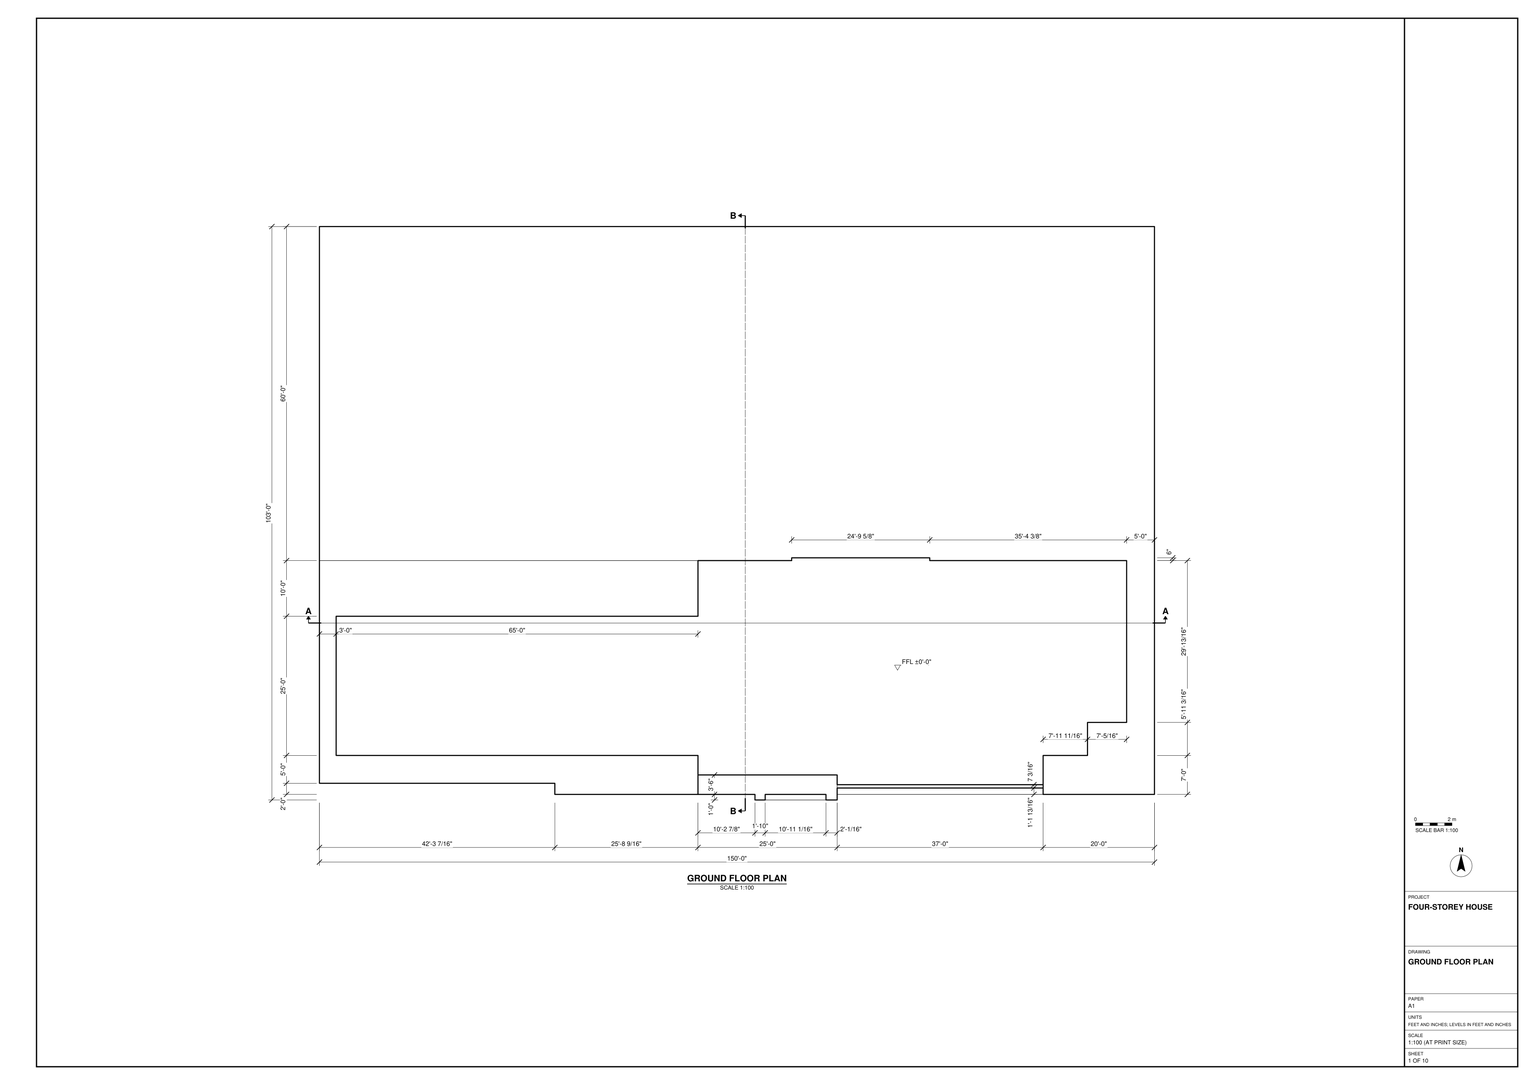
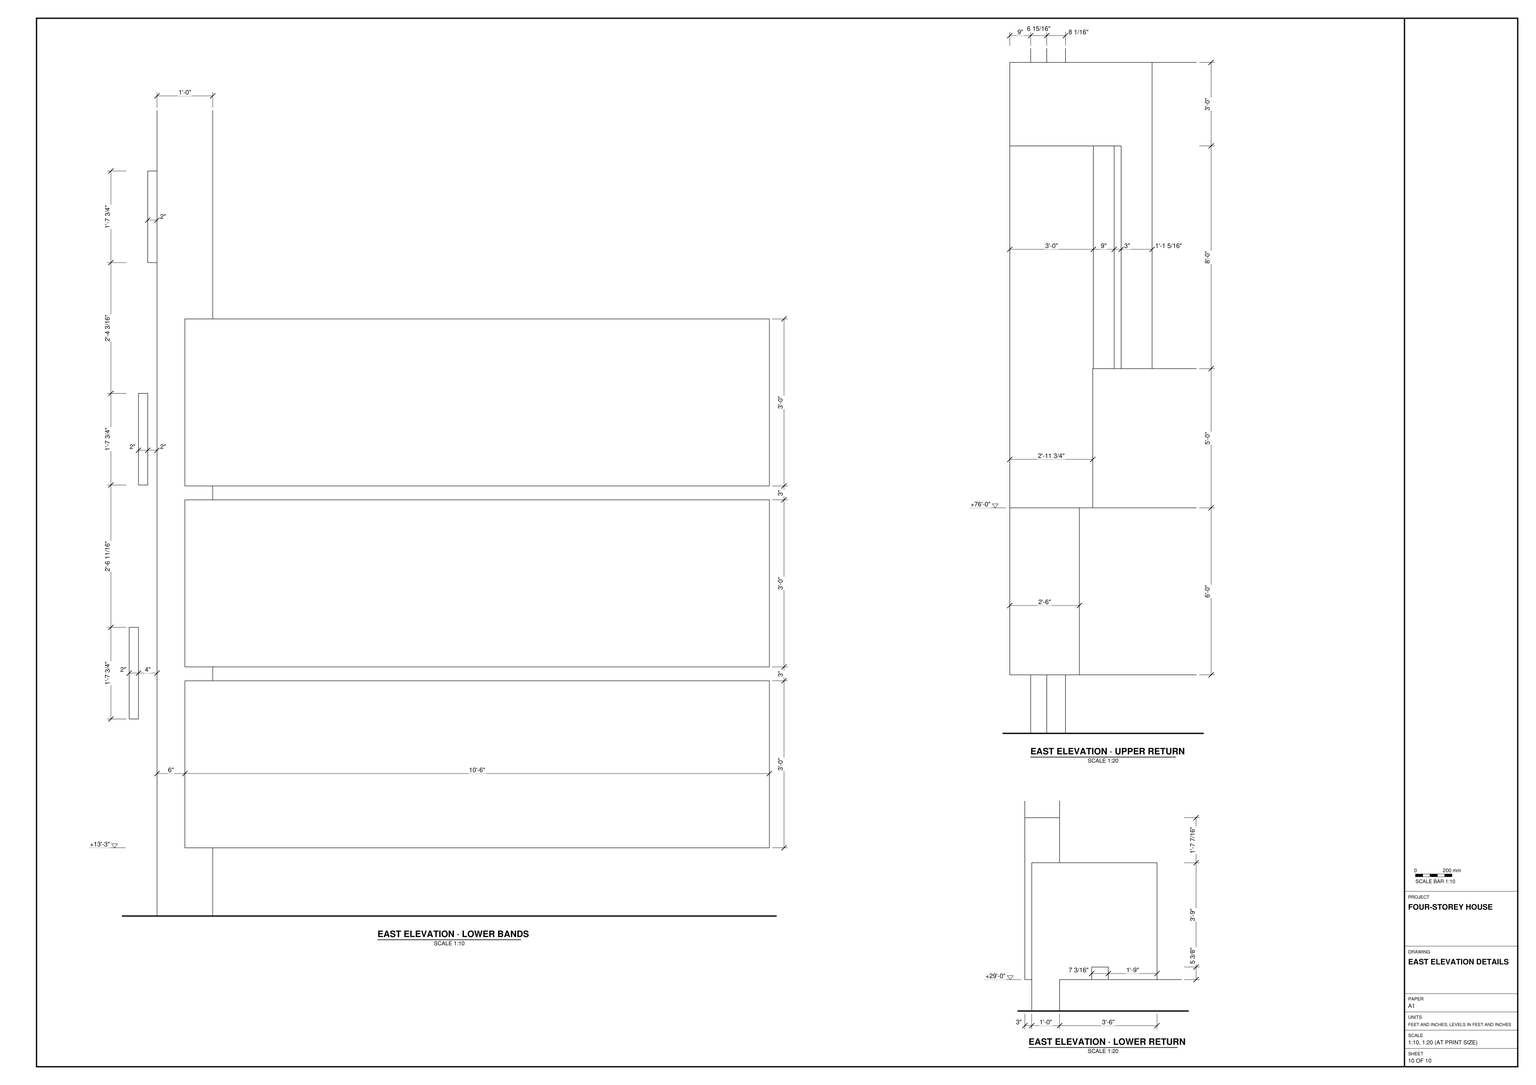
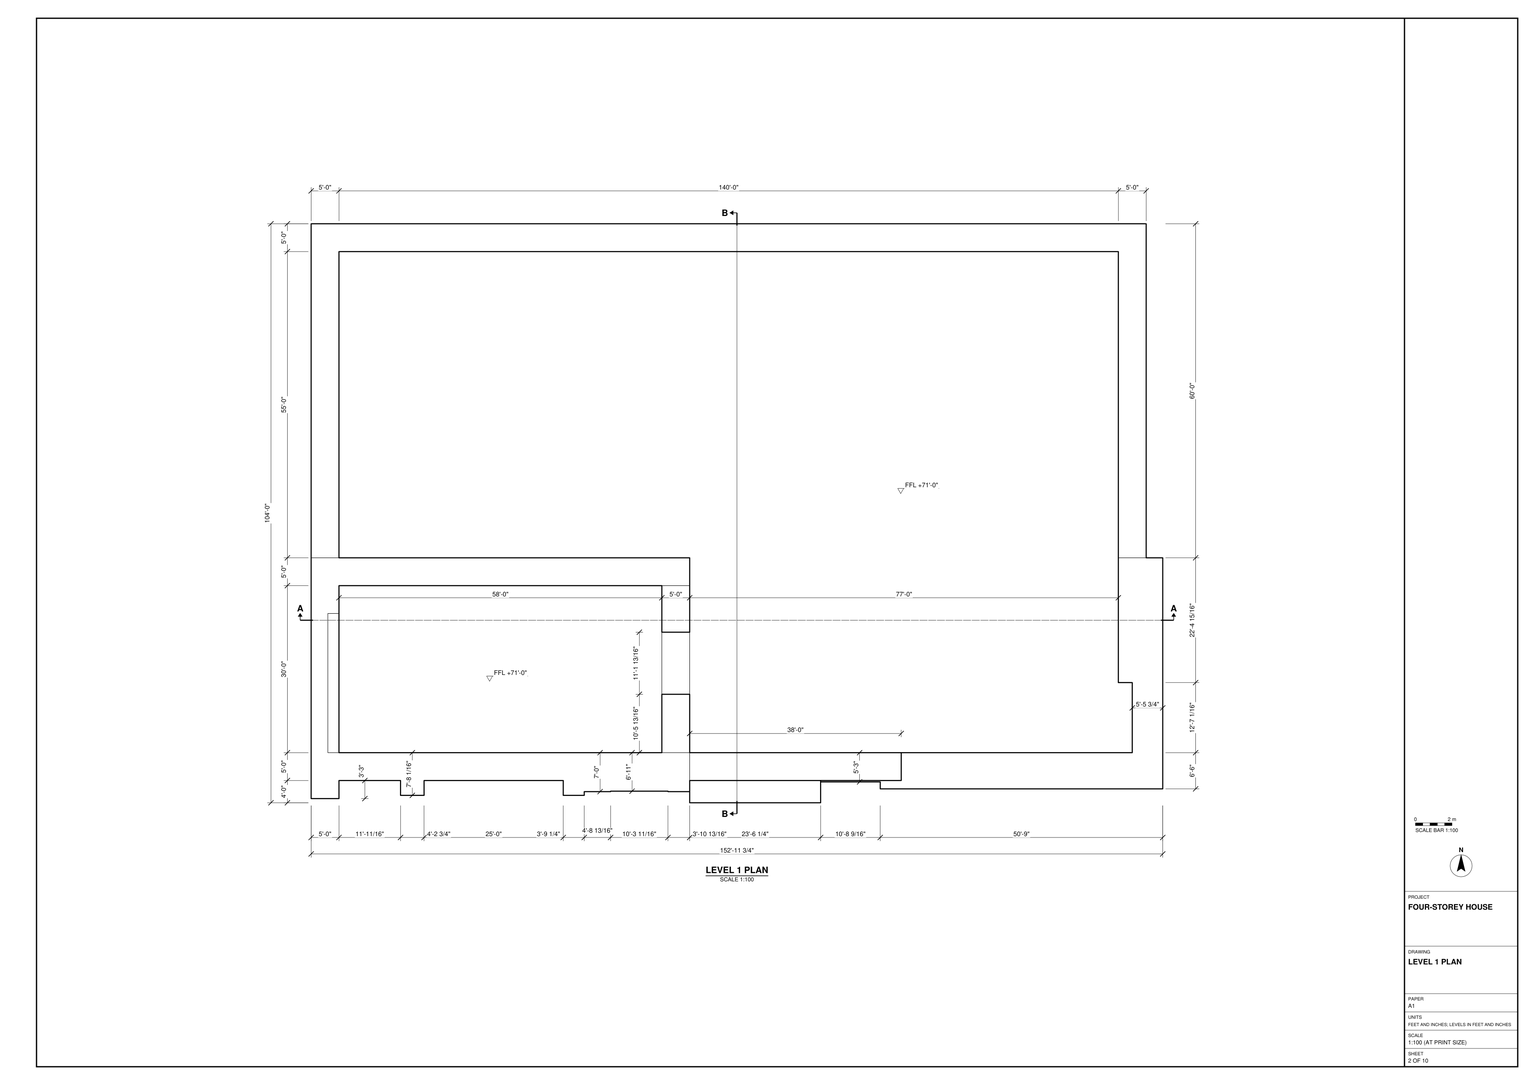
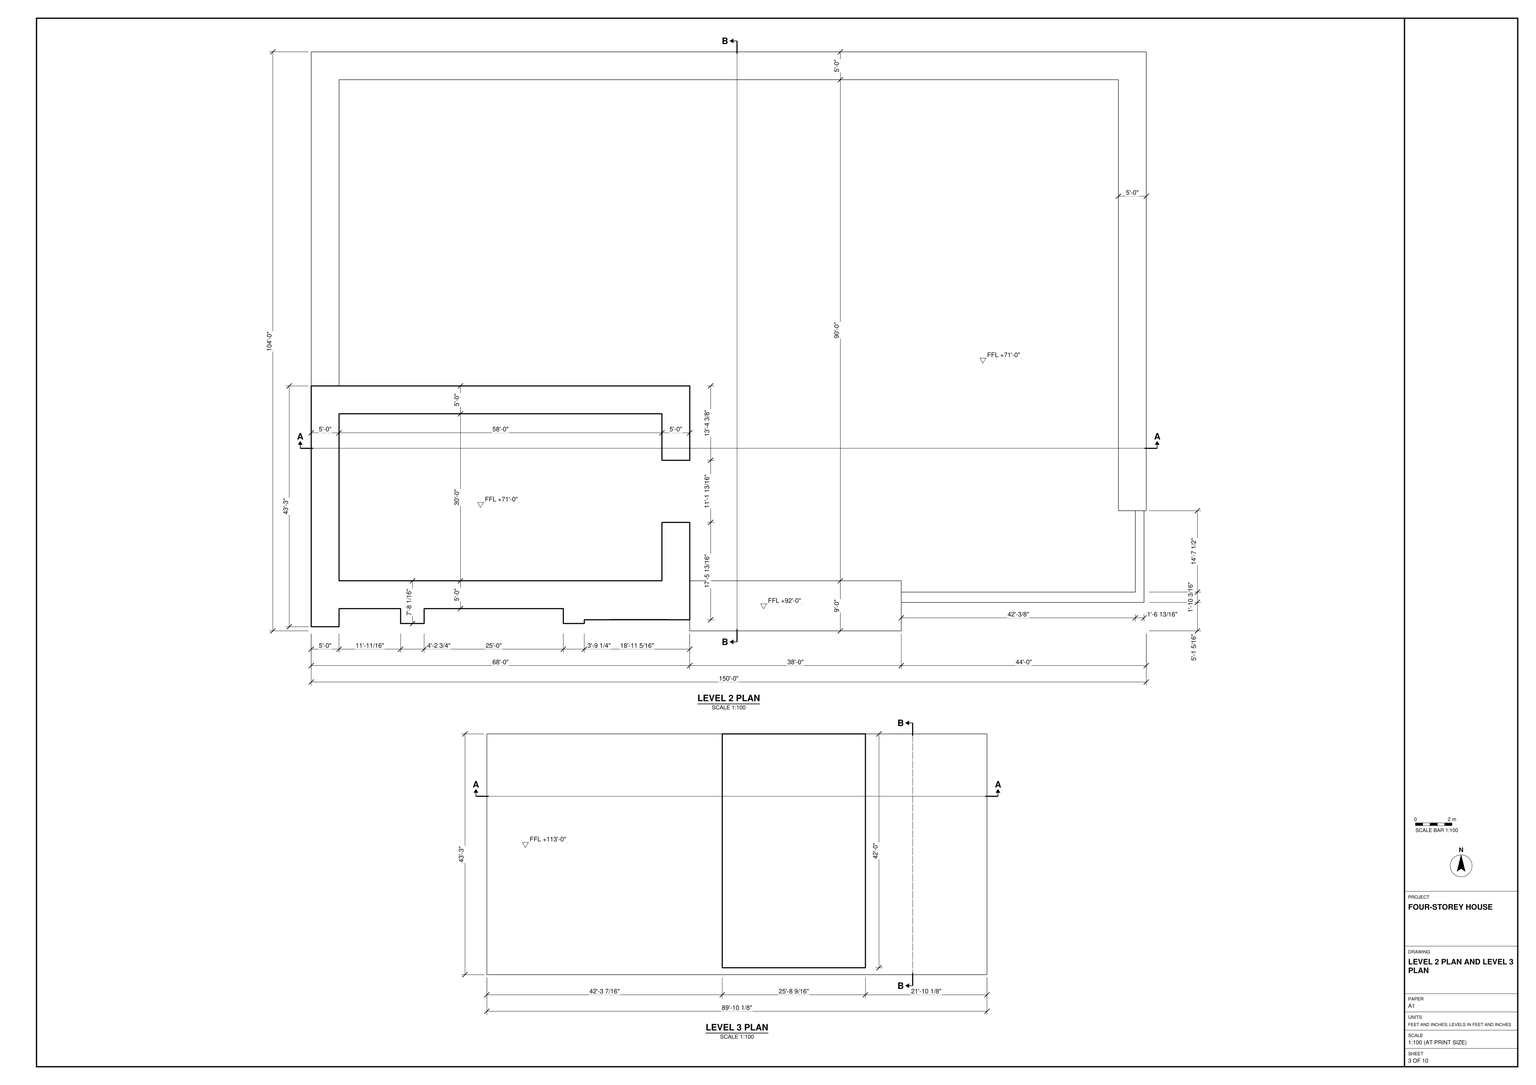
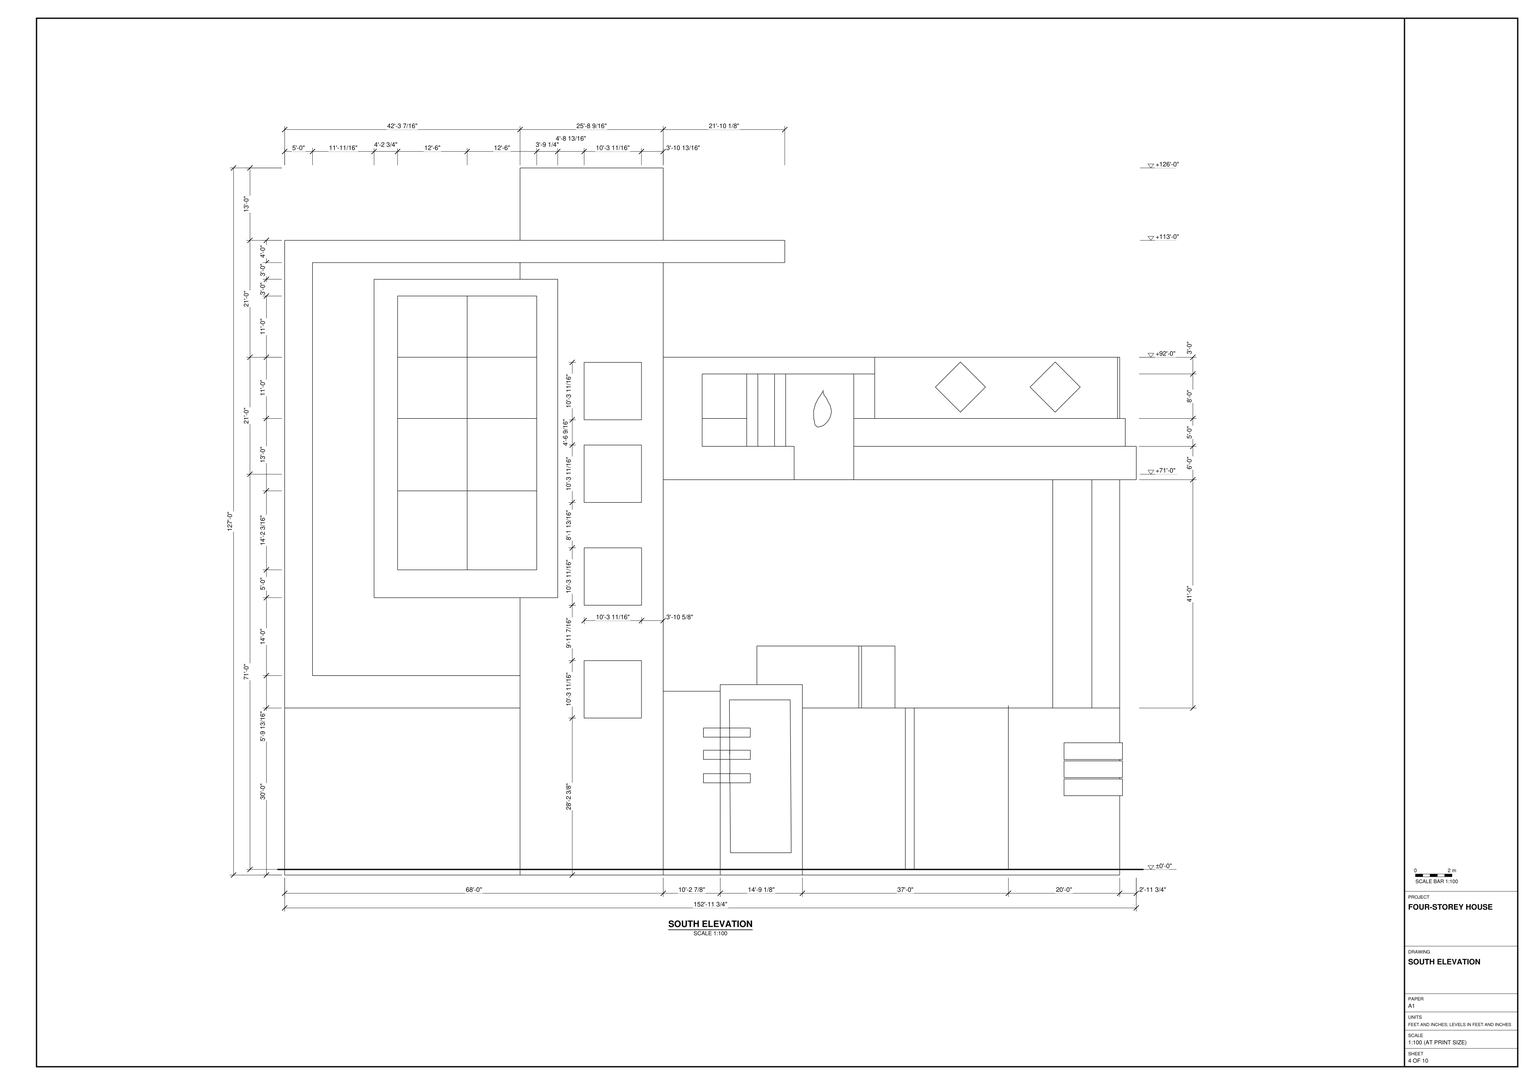
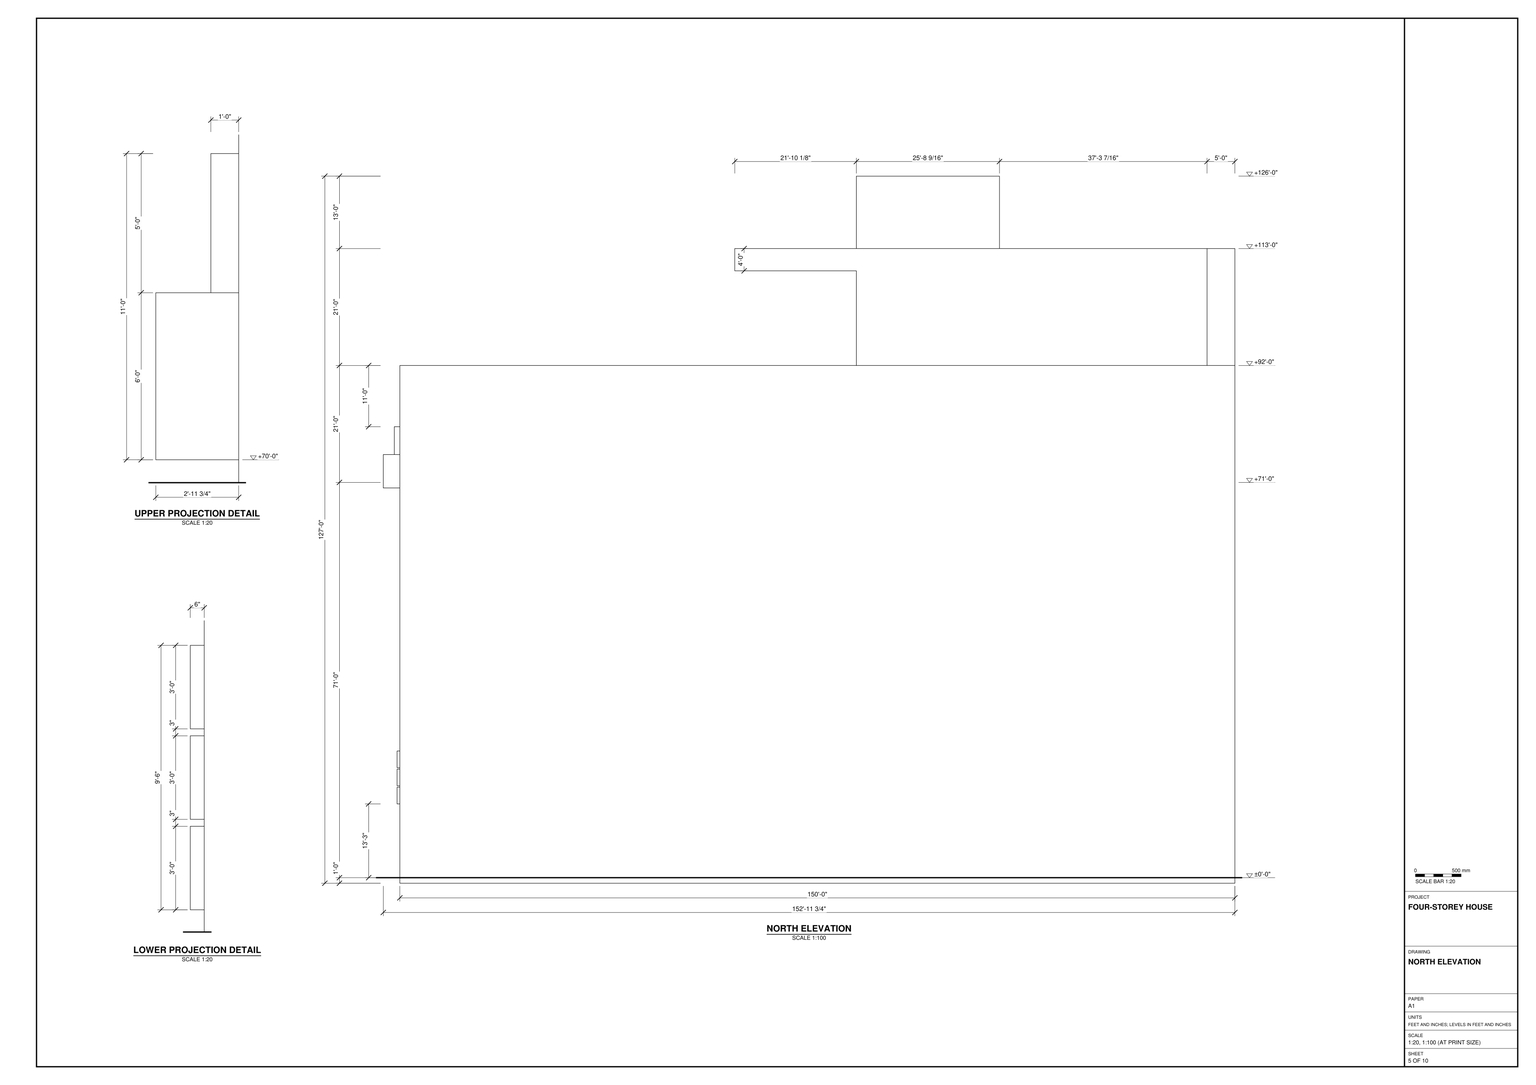
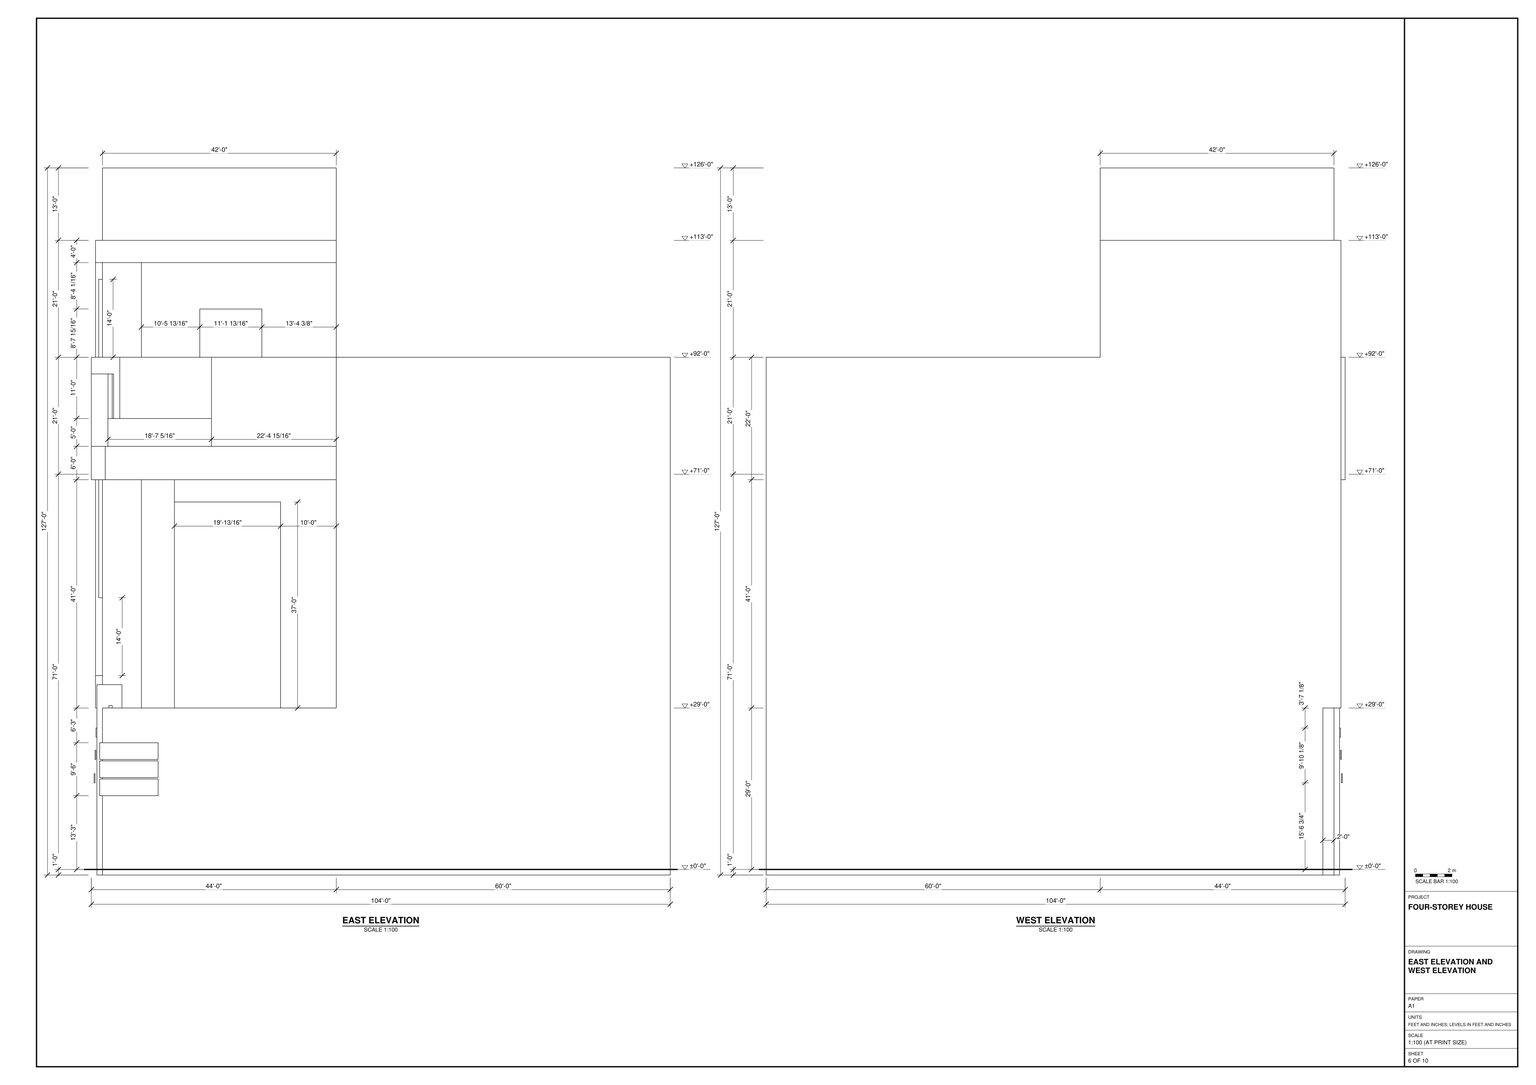
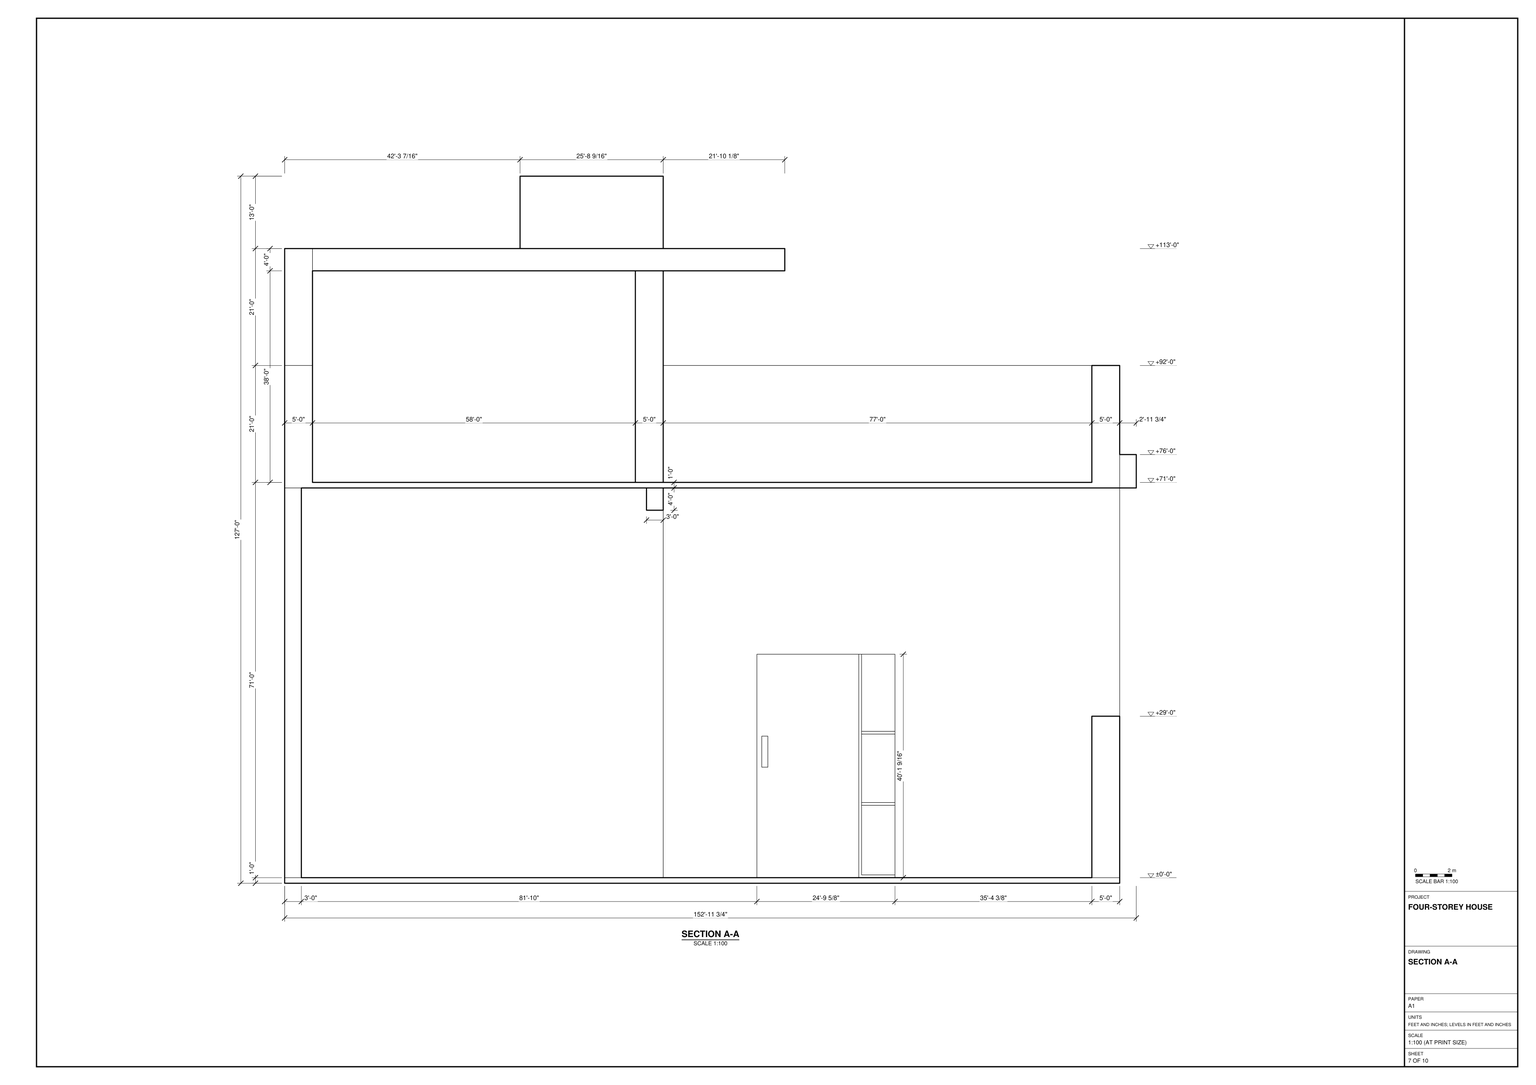
Build the four-storey house in SketchUp using task_files/diagram_01.pdf. Work in feet and inches. The overall model extents are 152'-11 3/4" along X, 104'-0" along Y and 127'-0" along Z. Set the ground floor at ±0'-0" and the three upper floor levels at +71'-0", +92'-0" and +113'-0".

Lay out each floor slab from its own plan. At the ground floor, follow the change in depth between the west and east portions and the stepped outline at the southeast corner. At the first upper level, preserve the relationship between the large L-shaped area and the smaller rectangular area to its southwest. Use the elevations and sections to set the wall profiles, slab edges and roof. Give the walls their drawn thicknesses and include the openings, stairs, built-in joinery and main furniture where shown. On the east elevation, model the three lower horizontal bands with the gaps between them, and follow the detail views for the profiles of the upper and lower returns.

Keep shell elements such as walls, slabs and roof in separate groups or components. Keep each furniture or joinery piece separate and use components for repeated parts. Any decor and loose items shown may be represented by suitable library components. Save one SketchUp model as output_files/four_storey_house_with_its_stepped_east_elevation.skp.

# SketchUp Ruby script. Lengths in inches.
U = 1.inch
M = Sketchup.active_model
def pt(a) = Geom::Point3d.new(a.map { |v| v * U })
def face(e, loops, mat)
  f = e.add_face(loops[0].map { |a| pt(a) })
  loops[1..].each { |l| e.add_face(l.map { |a| pt(a) }).erase! }
  f.material = f.back_material = mat if mat
  f
end
# faces: each face lists its corners as indices into pts; further lists are holes
def faces(e, pts, list, mat = nil) = list.each { |f| face(e, (f[0].is_a?(Array) ? f : [f]).map { |l| l.map { |i| pts[i] } }, mat) }
# xy, xz, yz: faces in a plane at the given z, y or x. An outline is a flat list of corners, or four numbers for a rectangle; further outlines are holes
def ring(l) = l.size == 4 ? [[l[0], l[1]], [l[2], l[1]], [l[2], l[3]], [l[0], l[3]]] : l.each_slice(2).to_a
def flat(e, list, mat, &to3) = list.each { |f| face(e, (f[0].is_a?(Array) ? f : [f]).map { |l| ring(l).map { |u, v| to3.(u, v) } }, mat) }
def xy(e, z, list, mat = nil) = flat(e, list, mat) { |x, y| [x, y, z] }
def xz(e, y, list, mat = nil) = flat(e, list, mat) { |x, z| [x, y, z] }
def yz(e, x, list, mat = nil) = flat(e, list, mat) { |y, z| [x, y, z] }
def lines(e, pts, list) = list.each { |a, b| e.add_line(pt(pts[a]), pt(pts[b])) }
# prism: a flat outline (further loops are holes) pulled along v
def prism(e, loops, v, mat = nil)
  f = face(e, loops, mat); d = Geom::Vector3d.new(v.map { |x| x * U })
  f.pushpull(f.normal.samedirection?(d) ? d.length : -d.length)
end
def box(e, o, s, mat = nil) = prism(e, [[o, [o[0] + s[0], o[1], o[2]], [o[0] + s[0], o[1] + s[1], o[2]], [o[0], o[1] + s[1], o[2]]]], [0, 0, s[2]], mat)
def at(x, y, z, deg = 0) = Geom::Transformation.translation(pt([x, y, z])) * Geom::Transformation.rotation(ORIGIN, Z_AXIS, deg.degrees)
def axes(o, x, y, z) = Geom::Transformation.new([*x, 0, *y, 0, *z, 0, *pt(o).to_a, 1])
def part(name) = M.definitions.add(name)
# library, detail: a bought-in or finely detailed component or shape, given as its bounding box
def library(name, o, s) = part(name).tap { |d| box(d.entities, o, s) }
def detail(e, o, s) = box(e.add_group.entities, o, s)
def put(e, d, t, mat = nil) = e.add_instance(d, t).tap { |i| i.material = mat if mat }
def group(e, t, mat = nil) = e.add_group.tap { |g| g.transformation = t; g.material = mat if mat }.entities
root = M.entities
M.materials.add("[0026_LightSalmon]").color = [255, 160, 122]
M.materials.add("[0029_BlanchedAlmond]").color = [209, 192, 168]
M.materials.add("[0030_OldLace]").color = [253, 245, 230]
M.materials.add("[0047_Khaki]").color = [201, 193, 117]
M.materials.add("[0058_Olive]").color = [76, 76, 0]
M.materials.add("[0119_RosyBrown]").color = [76, 58, 58]
M.materials.add("[0136_Charcoal]").color = [35, 35, 35]
M.materials.add("[0137_Black]").color = [0, 0, 0]
M.materials.add("[Blacktop Old 01]").color = [132, 136, 139]
M.materials.add("[Cladding Siding Tan]").color = [165, 128, 97]
M.materials.add("[Granite Brown]").color = [126, 104, 91]
M.materials.add("[Stone Flagstone Ashlar]").color = [175, 116, 102]
M.materials.add("[Stone Marble]").color = [143, 138, 136]
M.materials.add("[Translucent Glass Blue]").color = [100, 149, 237]
M.materials["[Translucent Glass Blue]"].alpha = 0.5
M.materials.add("[Translucent Glass Gray]").color = [128, 128, 128]
M.materials["[Translucent Glass Gray]"].alpha = 0.5
xy(root,0,[[938.875,12,938.875,24,507.4375,24,507.4375,48,0,48,0,1248,1800,1248,1800,24,1116,24,1116,12]])
xy(root,12,[[1116,24,1560,37.83],[1116,37.83,1560,45]])
xy(root,12,[[1116,45,1560,45,1560,108,1655.6875,108,1655.6875,179.1875,1740,179.1875,1740,528,1315.61,528,1315.61,534,1017.99,534,1017.99,528,816,528,816,408,36,408,36,108,816,108,816,66,1116,66]],"[Granite Brown]")
xy(root,48,[[960.9375,12,1092,24]],"[Blacktop Old 01]")
xy(root,171,[[1680,18,1806,24],[1800,24,1806,144]],"[Blacktop Old 01]")
xy(root,198.76,[[902.7,6,938.875,8],[938.875,6,959.26,8],[959.26,6,1003.82,8]],"[0047_Khaki]")
xy(root,207,[[1680,18,1806,24],[1800,24,1806,144]],"[0058_Olive]")
xy(root,210,[[1680,18,1806,24],[1800,24,1806,144]],"[Blacktop Old 01]")
xy(root,218.51,[[1003.6875,6,1003.82,8]])
xy(root,218.51,[[902.7,6,938.875,8],[938.875,6,959.125,8],[959.26,6,1003.6875,8]],"[0047_Khaki]")
xy(root,246,[[1680,18,1806,24],[1800,24,1806,144]],"[0058_Olive]")
xy(root,249,[[1680,18,1800,24],[1800,18,1806,144]],"[Blacktop Old 01]")
xy(root,249.2,[[902.7,8,938.875,10],[938.875,8,959.26,10],[959.26,8,1003.82,10]],"[0047_Khaki]")
xy(root,268.95,[[1003.6875,8,1003.82,10]])
xy(root,268.95,[[902.7,8,938.875,10],[938.875,8,959.125,10],[959.26,8,1003.6875,10]],"[0047_Khaki]")
xy(root,285,[[1680,18,1800,24],[1800,18,1806,144]],"[0058_Olive]")
xy(root,297.14,[[902.7,10,938.875,12],[938.875,10,959.26,12],[959.26,10,1003.82,12]],"[0047_Khaki]")
xy(root,316.89,[[1003.6875,10,1003.82,12]])
xy(root,316.89,[[902.7,10,938.875,12],[938.875,10,959.125,12],[959.26,10,1003.6875,12]],"[0047_Khaki]")
xy(root,338.36,[[645.5,24,769.18,25]])
xy(root,360,[[0,9,507.4375,48],[1560,24,1800,24,1800,528,1740,528,1740,108,1560,108],[1116,37.83,1560,45]])
xy(root,377.47,[[958.72,12,1089.78,24]],"[Blacktop Old 01]")
xy(root,396,[[816,24,938.875,66]])
xy(root,410.375,[[938.875,12,1116,66]],"[0058_Olive]")
xy(root,429.79,[[60,9,507.4375,48]],"[Blacktop Old 01]")
xy(root,462.04,[[645.5,24,769.18,25]])
xy(root,493.57,[[1017.99,528,1315.61,534]],"[0136_Charcoal]")
xy(root,581.5,[[645.66,24,769.35,25]])
xy(root,597.79,[[192.6875,15.9375,192.6875,48,507.4375,48,507.4375,24,588.6875,24,588.6875,15.9375]],"[0058_Olive]")
xy(root,657.79,[[243.4375,15.9375,543.4375,48]],"[0058_Olive]")
xy(root,705.1875,[[645.66,24,769.35,25]])
xy(root,803.01,[[645.5,24,769.18,25]])
xy(root,804,[[780,108,816,408]],"[Stone Flagstone Ashlar]")
xy(root,852,[[[1226.76,30,1226.76,45,1098.22,45,1098.22,48,816,48,816,528,1835.75,528,1835.75,30],[1655.6875,108,1740,179.1875],[1024.9,157.24,1031.11,158.0625,1036.9,160.46,1041.87,164.27,1045.6875,169.24,1048.08,175.03,1048.9,181.24,1048.08,187.46,1045.6875,193.24,1041.87,198.21,1036.9,202.03,1031.11,204.43,1024.9,205.24,1018.69,204.43,1012.9,202.03,1007.93,198.21,1004.12,193.24,1001.72,187.46,1000.9,181.24,1001.72,175.03,1004.12,169.24,1007.93,164.27,1012.9,160.46,1018.69,158.0625],[1293.34,157.24,1299.55,158.0625,1305.34,160.46,1310.31,164.27,1314.125,169.24,1316.52,175.03,1317.34,181.24,1316.52,187.46,1314.125,193.24,1310.31,198.21,1305.34,202.03,1299.55,204.43,1293.34,205.24,1287.13,204.43,1281.34,202.03,1276.37,198.21,1272.56,193.24,1270.16,187.46,1269.34,181.24,1270.16,175.03,1272.56,169.24,1276.37,164.27,1281.34,160.46,1287.13,158.0625],[1510.65,157.24,1516.86,158.0625,1522.65,160.46,1527.62,164.27,1531.4375,169.24,1533.83,175.03,1534.65,181.24,1533.83,187.46,1531.4375,193.24,1527.62,198.21,1522.65,202.03,1516.86,204.43,1510.65,205.24,1504.44,204.43,1498.65,202.03,1493.68,198.21,1489.87,193.24,1487.47,187.46,1486.65,181.24,1487.47,175.03,1489.87,169.24,1493.68,164.27,1498.65,160.46,1504.44,158.0625]],[780,108,816,408],[1024.9,157.24,1018.69,158.0625,1012.9,160.46,1007.93,164.27,1004.12,169.24,1001.72,175.03,1000.9,181.24,1001.72,187.46,1004.12,193.24,1007.93,198.21,1012.9,202.03,1018.69,204.43,1024.9,205.24,1031.11,204.43,1036.9,202.03,1041.87,198.21,1045.6875,193.24,1048.08,187.46,1048.9,181.24,1048.08,175.03,1045.6875,169.24,1041.87,164.27,1036.9,160.46,1031.11,158.0625],[1293.34,157.24,1287.13,158.0625,1281.34,160.46,1276.37,164.27,1272.56,169.24,1270.16,175.03,1269.34,181.24,1270.16,187.46,1272.56,193.24,1276.37,198.21,1281.34,202.03,1287.13,204.43,1293.34,205.24,1299.55,204.43,1305.34,202.03,1310.31,198.21,1314.125,193.24,1316.52,187.46,1317.34,181.24,1316.52,175.03,1314.125,169.24,1310.31,164.27,1305.34,160.46,1299.55,158.0625],[1510.65,157.24,1504.44,158.0625,1498.65,160.46,1493.68,164.27,1489.87,169.24,1487.47,175.03,1486.65,181.24,1487.47,187.46,1489.87,193.24,1493.68,198.21,1498.65,202.03,1504.44,204.43,1510.65,205.24,1516.86,204.43,1522.65,202.03,1527.62,198.21,1531.4375,193.24,1533.83,187.46,1534.65,181.24,1533.83,175.03,1531.4375,169.24,1527.62,164.27,1522.65,160.46,1516.86,158.0625]])
xy(root,852,[[816,0,1098.22,48]],"[0047_Khaki]")
xy(root,852,[[36,108,780,408]],"[Stone Flagstone Ashlar]")
xy(root,864,[[816,48,1272,108],[60,108,756,468],[756,108,816,233.83],[756,233.83,816,367.65],[756,367.65,816,468]])
xy(root,864,[[816,108,1770,108,1770,259.04,1740,259.04,1740,1188,60,1188,60,528,816,528]],"[0029_BlanchedAlmond]")
xy(root,912,[[1272,48,1800,48,1800,259.04,1795.23,259.04,1795.23,61.34,1272,61.34]])
xy(root,912,[[1272,83.56,1776.4,83.56,1776.4,259.04,1770,259.04,1770,108,1272,108]],"[0029_BlanchedAlmond]")
xy(root,924,[[996,36,1020,48],[1056,36,1080,48],[1020,45,1056,48],[1080,45,1098.22,48],[900,48,996,48.5]])
xy(root,924,[[900,0,1098.22,0,1098.22,45,1080,45,1080,36,1056,36,1056,45,1020,45,1020,36,996,36,996,48,900,48],[1226.76,30,1835.75,30,1835.75,528,1800,528,1800,259.04,1812,259.04,1812,35.75,1226.76,35.75]],"[0047_Khaki]")
xy(root,926.7,[[645.5,24,769.18,25]])
xy(root,981.26,[[645.5,24,769.18,25]])
xy(root,984,[[900,48,996,48.5]])
xy(root,984,[[1226.76,35.75,1812,35.75,1812,259.04,1800,259.04,1800,48,1226.76,48]],"[0026_LightSalmon]")
xy(root,1080,[[996,36,1020,48],[1056,36,1080,48],[1020,45,1056,48],[1080,45,1226.76,48]])
xy(root,1080,[[900,0,900,48,996,48,996,36,1020,36,1020,45,1056,45,1056,36,1080,36,1080,45,1226.76,45,1226.76,48,1272,48,1272,0]],"[0047_Khaki]")
xy(root,1104.94,[[645.5,24,769.18,25]])
xy(root,1116,[[1272,61.34,1795.23,61.34,1795.23,259.04,1776.4,259.04,1776.4,83.56,1272,83.56],[1740,259.04,1800,259.04,1800,1248,0,1248,0,528,60,528,60,1188,1740,1188]],"[0029_BlanchedAlmond]")
xy(root,1116,[[816,0,1272,108]],"[0047_Khaki]")
xy(root,1219.9375,[[756,233.83,816,367.65]])
xy(root,1248,[[243.4375,15.9375,543.4375,48]],"[0058_Olive]")
xy(root,1284,[[192.6875,15.9375,588.6875,15.9375,588.6875,24,507.4375,24,507.4375,48,192.6875,48]],"[0058_Olive]")
xy(root,1320,[[[816,9,1078.125,108],[966.1,34.06,972.25,35.25,977.89,37.99,982.62,42.09,986.13,47.28,988.18,53.2,988.62,59.45,987.43,65.6,984.69,71.24,980.59,75.97,975.4,79.48,969.48,81.53,963.23,81.97,957.08,80.78,951.44,78.04,946.71,73.9375,943.2,68.75,941.15,62.83,940.71,56.58,941.9,50.43,944.64,44.79,948.74,40.06,953.93,36.55,959.85,34.5]],[966.1,34.06,959.85,34.5,953.93,36.55,948.74,40.06,944.64,44.79,941.9,50.43,940.71,56.58,941.15,62.83,943.2,68.75,946.71,73.9375,951.44,78.04,957.08,80.78,963.23,81.97,969.48,81.53,975.4,79.48,980.59,75.97,984.69,71.24,987.43,65.6,988.62,59.45,988.18,53.2,986.13,47.28,982.62,42.09,977.89,37.99,972.25,35.25],[60,108,756,468],[756,108,816,468],[[816,108,1078.125,468],[844.55,155.55,1032.24,184.18],[844.55,222.55,1032.24,251.18],[844.55,284.61,1032.24,313.24],[844.55,347.05,1032.24,375.68],[844.55,410.43,1032.24,439.05]],
  [[816,468,1078.125,528],[966.1,475.68,972.25,476.87,977.89,479.61,982.62,483.71,986.13,488.9,988.18,494.83,988.62,501.08,987.43,507.23,984.69,512.86,980.59,517.6,975.4,521.1,969.48,523.15,963.23,523.6,957.08,522.41,951.44,519.67,946.71,515.5625,943.2,510.375,941.15,504.45,940.71,498.2,941.9,492.05,944.64,486.42,948.74,481.68,953.93,478.17,959.85,476.125]],[966.1,475.68,959.85,476.125,953.93,478.17,948.74,481.68,944.64,486.42,941.9,492.05,940.71,498.2,941.15,504.45,943.2,510.375,946.71,515.5625,951.44,519.67,957.08,522.41,963.23,523.6,969.48,523.15,975.4,521.1,980.59,517.6,984.69,512.86,987.43,507.23,988.62,501.08,988.18,494.83,986.13,488.9,982.62,483.71,977.89,479.61,972.25,476.87]])
xy(root,1320,[[844.55,155.55,1032.24,184.18],[844.55,222.55,1032.24,251.18],[844.55,284.61,1032.24,313.24],[844.55,347.05,1032.24,375.68],[844.55,410.43,1032.24,439.05]],"[0058_Olive]")
xy(root,1320,[[60,9,60,48,507.4375,48,507.4375,24,816,24,816,9]],"[Blacktop Old 01]")
xy(root,1368,[[507.4375,24,816,528]])
xy(root,1368,[[0,9,1078.125,9,1078.125,528,816,528,816,24,507.4375,24,507.4375,528,0,528]],"[0029_BlanchedAlmond]")
xy(root,1524,[[507.4375,24,816,528]],"[Stone Flagstone Ashlar]")
xz(root,0,[[816,852,1098.22,852,1098.22,924,900,924,900,1080,1272,1080,1272,1116,816,1116]],"[0047_Khaki]")
xz(root,6,[[902.7,198.76,938.875,218.51],[938.875,198.76,959.26,198.76,959.125,218.51,938.875,218.51],[959.26,198.76,1003.82,218.51]],"[0047_Khaki]")
xz(root,8,[[902.7,198.76,938.875,218.51],[938.875,198.76,938.875,218.51,959.125,218.51,959.26,198.76],[959.26,198.76,1003.82,218.51]])
xz(root,8,[[902.7,249.2,938.875,268.95],[938.875,249.2,959.26,249.2,959.125,268.95,938.875,268.95],[959.26,249.2,1003.82,268.95]],"[0047_Khaki]")
xz(root,9,[[0,360,507.4375,360,507.4375,429.79,60,429.79,60,1320,1078.125,1320,1078.125,1368,0,1368]],"[Blacktop Old 01]")
xz(root,10,[[902.7,249.2,938.875,268.95],[938.875,249.2,938.875,268.95,959.125,268.95,959.26,249.2],[959.26,249.2,1003.82,268.95]])
xz(root,10,[[902.7,297.14,938.875,316.89],[938.875,297.14,959.26,297.14,959.125,316.89,938.875,316.89],[959.26,297.14,1003.82,316.89]],"[0047_Khaki]")
xz(root,12,[[902.7,297.14,938.875,316.89],[938.875,297.14,938.875,316.89,959.125,316.89,959.26,297.14],[959.26,297.14,959.26,316.89,959.125,316.89],[959.26,297.14,1003.82,316.89]])
xz(root,12,[[938.875,0,1116,0,1116,410.375,938.875,410.375,938.875,316.89,959.125,316.89,958.72,377.47,1089.78,377.47,1092,48,960.9375,48,959.26,297.14,938.875,297.14]],"[0058_Olive]")
xz(root,15.9375,[[[192.6875,597.79,588.6875,1284],[243.4375,657.79,543.4375,1248]]],"[0058_Olive]")
xz(root,18,[[1680,171,1806,207],[1680,210,1806,246],[1680,249,1806,285]],"[0058_Olive]")
xz(root,24,[[1680,249,1800,285]])
xz(root,24,[[816,0,938.875,12],[1116,0,1800,0,1800,171,1680,171,1680,207,1800,207,1800,210,1680,210,1680,246,1800,246,1800,249,1680,249,1680,285,1800,285,1800,360,1560,360,1560,12,1116,12],[816,12,938.875,396],[960.9375,48,1092,48,1089.78,377.47,958.72,377.47]],"[0029_BlanchedAlmond]")
xz(root,24,[[[507.4375,0,816,0,816,1320,507.4375,1320,507.4375,1284,588.6875,1284,588.6875,597.79,507.4375,597.79],[645.5,803.01,769.18,926.7],[645.66,581.5,769.35,705.1875],[645.5,338.36,769.18,462.04],[645.5,981.26,769.18,1104.94]],[507.4375,1368,816,1524]],"[Stone Flagstone Ashlar]")
xz(root,25,[[645.5,338.36,769.18,462.04],[645.66,581.5,769.35,705.1875],[645.5,803.01,769.18,926.7],[645.5,981.26,769.18,1104.94]])
xz(root,30,[[1226.76,852,1835.75,924]],"[0047_Khaki]")
xz(root,35.75,[[1226.76,924,1812,984]],"[0026_LightSalmon]")
xz(root,36,[[996,924,1020,1080],[1056,924,1080,1080]],"[0058_Olive]")
xz(root,37.83,[[1338,12,1357.125,360]],"[0137_Black]")
xz(root,37.83,[[1116,12,1338,360],[1357.125,12,1560,360]],"[Cladding Siding Tan]")
xz(root,45,[[1116,12,1560,360]])
xz(root,45,[[1020,924,1056,1080]],"[0029_BlanchedAlmond]")
xz(root,45,[[1148.98,965.29,1155.99,967.1,1159.14,968,1161.29,969.05,1163.43,970.8,1165.51,972.6,1167.52,974.44,1169.45,976.36,1171.03,978.63,1172.54,980.9,1173.95,983.2,1175.28,985.55,1176.2,987.91,1176.81,990.32,1177.62,993.31,1178.04,995.625,1178.57,997.98,1178.4375,1000.625,1178.18,1003,1177.33,1005.38,1176.97,1007.82,1176.23,1010.83,1175.34,1013.21,1173.89,1015.58,1172.59,1018.22,1170.78,1021.1,1170.22,1022.86,1167.6,1028.03,1162.8,1034.4,1160.35,1042.71,1159.09,1040.51,1157.58,1038.3,1156.34,1036.12,1154.82,1034.24,1153.85,1031.96,1152.26,1029.73,1150.73,1027.74,1149.25,1025.13,1148.08,1022.85,1146.98,1020.57,1145.85,1018.28,1144.28,1015.97,1143.94,1013.61,1142.99,1011.24,1142.36,1008.81,1141.77,1006.06,1140.9375,1003.62,1140.24,1000.85,1140.22,998.1,1140.21,995.65,1140.22,992.88,1140.25,990.16,1140.37,987.71,1140.54,984.95,1140.73,982.53,1141.62,979.57,1142.25,976.86,1142,974.92,1143.57,969.82]],"[0030_OldLace]")
xz(root,45,[[[1098.22,852,1226.76,852,1226.76,1080,1080,1080,1080,924,1098.22,924],[1148.98,965.29,1143.57,969.82,1142,974.92,1142.25,976.86,1141.62,979.57,1140.73,982.53,1140.54,984.95,1140.37,987.71,1140.25,990.16,1140.22,992.88,1140.21,995.65,1140.22,998.1,1140.24,1000.85,1140.9375,1003.62,1141.77,1006.06,1142.36,1008.81,1142.99,1011.24,1143.94,1013.61,1144.28,1015.97,1145.85,1018.28,1146.98,1020.57,1148.08,1022.85,1149.25,1025.13,1150.73,1027.74,1152.26,1029.73,1153.85,1031.96,1154.82,1034.24,1156.34,1036.12,1157.58,1038.3,1159.09,1040.51,1160.35,1042.71,1162.8,1034.4,1167.6,1028.03,1170.22,1022.86,1170.78,1021.1,1172.59,1018.22,1173.89,1015.58,1175.34,1013.21,1176.23,1010.83,1176.97,1007.82,1177.33,1005.38,1178.18,1003,1178.4375,1000.625,1178.57,997.98,1178.04,995.625,1177.62,993.31,1176.81,990.32,1176.2,987.91,1175.28,985.55,1173.95,983.2,1172.54,980.9,1171.03,978.63,1169.45,976.36,1167.52,974.44,1165.51,972.6,1163.43,970.8,1161.29,969.05,1159.14,968,1155.99,967.1]]],"[0058_Olive]")
xz(root,48,[[816,864,1098.22,864,1098.22,924,900,924,900,984,816,984],[1098.22,864,1272,864,1272,984,996,984,996,924,1098.22,924],[1272,912,1800,984]])
xz(root,48,[[60,429.79,507.4375,429.79,507.4375,597.79,192.6875,597.79,192.6875,1284,507.4375,1284,507.4375,1320,60,1320],[900,924,996,984],[900,984,996,1080],[1226.76,984,1272,1080]],"[0029_BlanchedAlmond]")
xz(root,48,[[0,0,507.4375,360]],"[0047_Khaki]")
xz(root,48,[[243.4375,657.79,393.4375,828],[393.4375,657.79,543.4375,828],[243.4375,828,393.4375,984],[393.4375,828,543.4375,984],[243.4375,984,393.4375,1116],
  [393.4375,984,543.4375,1116],[243.4375,1116,393.4375,1248],[393.4375,1116,543.4375,1248]],"[Translucent Glass Blue]")
xz(root,48.5,[[900,924,996,984]])
xz(root,61.34,[[[1272,912,1795.23,1116],[1660.89,997.66,1606.84,1051.71,1660.89,1105.76,1714.9375,1051.71],[1456.7,997.66,1402.65,1051.71,1456.7,1105.76,1510.75,1051.71]]],"[0029_BlanchedAlmond]")
xz(root,66,[[816,12,816,396,938.875,396,938.875,410.375,1116,410.375,1116,12]],"[0058_Olive]")
xz(root,73.34,[[1456.7,997.66,1510.75,1051.71,1456.7,1105.76,1402.65,1051.71],[1660.89,997.66,1714.9375,1051.71,1660.89,1105.76,1606.84,1051.71]],"[0058_Olive]")
xz(root,83.56,[[1272,912,1776.4,1116]],"[0029_BlanchedAlmond]")
xz(root,108,[[1560,12,1655.6875,360],[60,864,756,1320]])
xz(root,108,[[1272,864,1770,912]],"[0029_BlanchedAlmond]")
xz(root,108,[[816,864,1272,1116]],"[0047_Khaki]")
xz(root,108,[[36,12,36,852,780,852,780,804,816,804,816,12],[1655.6875,360,1740,852]],"[Stone Flagstone Ashlar]")
xz(root,144,[[1800,171,1806,207],[1800,210,1806,246],[1800,249,1806,285]],"[0058_Olive]")
xz(root,179.1875,[[1655.6875,12,1740,852]],"[Stone Flagstone Ashlar]")
xz(root,233.83,[[756,864,816,1219.9375]],"[0026_LightSalmon]")
xz(root,259.04,[[1795.23,912,1800,1116]])
xz(root,259.04,[[1800,924,1812,984]],"[0026_LightSalmon]")
xz(root,259.04,[[1740,864,1770,864,1770,912,1776.4,912,1776.4,1116,1740,1116]],"[0029_BlanchedAlmond]")
xz(root,367.65,[[756,864,816,1219.9375]],"[0026_LightSalmon]")
xz(root,408,[[36,12,816,12,816,804,780,804,780,852,36,852]],"[Stone Flagstone Ashlar]")
xz(root,468,[[60,864,756,1320]])
xz(root,528,[[60,864,60,1368,1078.125,1368,1078.125,1320,816,1320,816,864],[0,1116,60,1368]],"[0029_BlanchedAlmond]")
xz(root,528,[[1800,852,1835.75,924]],"[0047_Khaki]")
xz(root,528,[[507.4375,1368,816,1524]],"[Stone Flagstone Ashlar]")
xz(root,528,[[816,12,1017.99,12,1017.99,493.57,1315.61,493.57,1315.61,12,1740,12,1740,360,1800,360,1800,852,816,852]],"[Stone Marble]")
xz(root,534,[[1028.48,250.13,1041.6,317.07]])
xz(root,534,[[[1017.99,12,1237.61,493.57],[1028.48,250.13,1041.6,317.07]]],"[0119_RosyBrown]")
xz(root,534,[[1237.61,12,1315.61,12,1315.61,18,1243.61,18,1243.61,493.57,1237.61,493.57],[1243.61,168,1315.61,174],[1243.61,321.4375,1315.61,327.4375]],"[0136_Charcoal]")
xz(root,534,[[1243.61,18,1315.61,168],[1243.61,174,1315.61,321.4375],[1243.61,327.4375,1315.61,493.57]],"[Translucent Glass Gray]")
xz(root,1188,[[60,864,1740,1116]],"[0029_BlanchedAlmond]")
xz(root,1248,[[0,0,1800,12],[0,12,1800,1116]])
yz(root,0,[[48,0,48,360,9,360,9,1368,528,1368,528,1116,1248,1116,1248,0]],"[0029_BlanchedAlmond]")
yz(root,36,[[108,12,408,852]],"[Stone Flagstone Ashlar]")
yz(root,60,[[108,864,468,1320],[528,864,1188,1116]])
yz(root,60,[[9,429.79,48,1320]],"[Blacktop Old 01]")
yz(root,192.6875,[[15.9375,597.79,48,1284]],"[0058_Olive]")
yz(root,243.4375,[[15.9375,657.79,48,1248]],"[0058_Olive]")
yz(root,507.4375,[[24,360,48,429.79]])
yz(root,507.4375,[[9,360,24,429.79]],"[Blacktop Old 01]")
yz(root,507.4375,[[24,0,48,360],[24,429.79,48,597.79],[24,1284,48,1320],[24,1368,528,1524]],"[Stone Flagstone Ashlar]")
yz(root,543.4375,[[15.9375,657.79,48,1248]],"[0058_Olive]")
yz(root,588.6875,[[15.9375,597.79,24,1284]],"[0058_Olive]")
yz(root,645.5,[[24,338.36,25,462.04],[24,803.01,25,926.7],[24,981.26,25,1104.94]])
yz(root,645.66,[[24,581.5,25,705.1875]])
yz(root,756,[[108,864,108,1320,468,1320,468,864,367.65,864,367.65,1219.9375,233.83,1219.9375,233.83,864]])
yz(root,769.18,[[24,338.36,25,462.04],[24,803.01,25,926.7],[24,981.26,25,1104.94]])
yz(root,769.35,[[24,581.5,25,705.1875]])
yz(root,780,[[108,804,408,852]])
yz(root,816,[[24,12,66,396],[24,852,48,1116]])
yz(root,816,[[108,864,233.83,864,233.83,1219.9375,367.65,1219.9375,367.65,864,528,864,528,1320,108,1320]],"[0026_LightSalmon]")
yz(root,816,[[0,852,24,1116]],"[0047_Khaki]")
yz(root,816,[[66,12,108,12,108,804,408,804,408,12,528,12,528,852,24,852,24,396,66,396],[24,1116,108,1320],[24,1368,528,1524]],"[Stone Flagstone Ashlar]")
yz(root,900,[[48,924,48.5,984]])
yz(root,900,[[0,924,48,1080]],"[0047_Khaki]")
yz(root,902.7,[[6,198.76,8,218.51],[8,249.2,10,268.95],[10,297.14,12,316.89]],"[0047_Khaki]")
yz(root,938.875,[[6,198.76,8,218.51],[8,249.2,10,268.95],[10,297.14,12,316.89]])
yz(root,938.875,[[12,0,24,12],[12,12,24,396],[12,396,66,410.375]],"[Blacktop Old 01]")
yz(root,959.26,[[6,198.76,8,218.51],[8,249.2,10,268.95],[10,297.14,12,316.89]])
yz(root,996,[[48,924,48.5,984]])
yz(root,996,[[36,924,48,1080]],"[0058_Olive]")
yz(root,1003.82,[[6,198.76,8,218.51],[8,249.2,10,268.95],[10,297.14,12,316.89]],"[0047_Khaki]")
yz(root,1017.99,[[528,12,534,493.57]],"[0136_Charcoal]")
yz(root,1020,[[36,924,45,1080]],"[0058_Olive]")
yz(root,1056,[[36,924,45,1080]],"[0058_Olive]")
yz(root,1078.125,[[9,1320,528,1368]])
yz(root,1080,[[36,924,45,1080]],"[0058_Olive]")
yz(root,1098.22,[[45,852,48,924]])
yz(root,1098.22,[[0,852,45,924]],"[0047_Khaki]")
yz(root,1116,[[12,0,24,0,24,12,37.83,12,37.83,365.4,45,365.4,45,12,66,12,66,410.375,12,410.375]],"[0058_Olive]")
yz(root,1116,[[37.83,360,45,365.4]],"[Blacktop Old 01]")
yz(root,1226.76,[[30,852,45,924],[35.75,924,45,984]],"[0047_Khaki]")
yz(root,1226.76,[[45,984,48,1080]],"[0058_Olive]")
yz(root,1272,[[48,864,108,864,108,912,83.56,912,83.56,1116,61.34,1116,61.34,912,48,912]])
yz(root,1272,[[48,912,61.34,912,61.34,1116,0,1116,0,1080,48,1080],[83.56,912,108,1116]],"[0047_Khaki]")
yz(root,1315.61,[[528,12,534,493.57]],"[0136_Charcoal]")
yz(root,1560,[[24,12,37.83,360],[37.83,12,45,360],[45,12,108,360],[37.83,360,45,365.4]])
yz(root,1655.6875,[[108,12,179.1875,852]],"[Stone Flagstone Ashlar]")
yz(root,1680,[[18,171,24,207],[18,210,24,246],[18,249,24,285]],"[0058_Olive]")
yz(root,1740,[[179.1875,12,528,360]])
yz(root,1740,[[259.04,864,1188,1116]],"[0029_BlanchedAlmond]")
yz(root,1740,[[108,360,179.1875,852]],"[Stone Flagstone Ashlar]")
yz(root,1770,[[108,864,259.04,912]],"[0029_BlanchedAlmond]")
yz(root,1776.4,[[83.56,912,259.04,1116]],"[0029_BlanchedAlmond]")
yz(root,1795.23,[[61.34,912,259.04,1116]],"[0029_BlanchedAlmond]")
yz(root,1800,[[48,912,259.04,984]])
yz(root,1800,[[24,0,1248,0,1248,1116,528,1116,528,360,24,360,24,285,144,285,144,249,24,249,24,246,144,246,144,210,24,210,24,207,144,207,144,171,24,171],[259.04,924,528,1116]],"[0029_BlanchedAlmond]")
yz(root,1806,[[18,171,144,207],[18,210,144,246],[18,249,144,285]],"[0058_Olive]")
yz(root,1812,[[35.75,924,259.04,984]],"[0026_LightSalmon]")
yz(root,1835.75,[[30,852,528,924]],"[0047_Khaki]")
p = [[960.9375,24,48],[958.72,24,377.47],[958.72,12,377.47],[959.125,12,316.89],[959.26,12,297.14],[960.9375,12,48],
  [1089.78,24,377.47],[1092,24,48],[1092,12,48],[1089.78,12,377.47],[959.26,8,198.76],[959.125,8,218.51],
  [959.125,6,218.51],[959.26,6,198.76],[959.26,10,249.2],[959.125,10,268.95],[959.125,8,268.95],[959.26,8,249.2],
  [959.125,10,316.89],[959.26,10,297.14],[1402.65,61.34,1051.71],[1456.7,61.34,997.66],[1456.7,73.34,997.66],[1402.65,73.34,1051.71],
  [1510.75,61.34,1051.71],[1510.75,73.34,1051.71],[1606.84,61.34,1051.71],[1660.89,61.34,997.66],[1660.89,73.34,997.66],[1606.84,73.34,1051.71],
  [1714.9375,61.34,1051.71],[1714.9375,73.34,1051.71],[1456.7,61.34,1105.76],[1456.7,73.34,1105.76],[1660.89,61.34,1105.76],[1660.89,73.34,1105.76],
  [60,108,1320],[60,108,1368],[60,468,1320],[60,468,1368],[1160.35,45,1042.71],[1161.56,45,1044.95],
  [816,48,1320],[816,48,1368],[816,108,984],[816,48,984],[816,528,12],[0,528,12],
  [816,528,852],[0,528,852]]
faces(root,p,[[0,1,2,3,4,5],[20,21,22,23],[21,24,25,22],[26,27,28,29],[27,30,31,28],[32,20,23,33],[24,32,33,25],[34,26,29,35],
  [30,34,35,31]],"[0058_Olive]")
faces(root,p,[[6,7,8,9]],"[Blacktop Old 01]")
faces(root,p,[[10,11,12,13],[14,15,16,17],[4,3,18,19]])
lines(root,p,[[36,37],[38,39],[40,41],[42,43],[44,45],[46,47],[48,49]])
